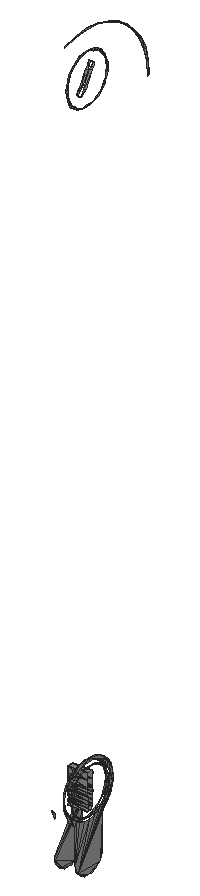
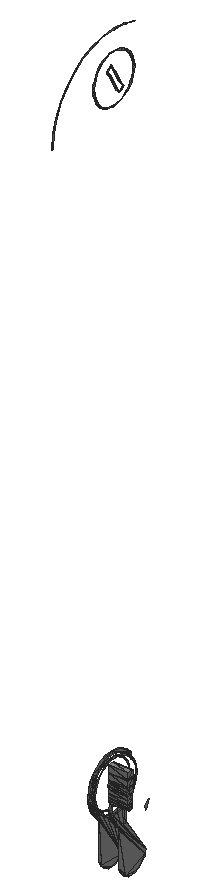
# SketchUp Ruby script. Lengths in inches.
U = 1.inch
M = Sketchup.active_model
def pt(a) = Geom::Point3d.new(a.map { |v| v * U })
def face(e, loops, mat)
  f = e.add_face(loops[0].map { |a| pt(a) })
  loops[1..].each { |l| e.add_face(l.map { |a| pt(a) }).erase! }
  f.material = f.back_material = mat if mat
  f
end
# faces: each face lists its corners as indices into pts; further lists are holes
def faces(e, pts, list, mat = nil) = list.each { |f| face(e, (f[0].is_a?(Array) ? f : [f]).map { |l| l.map { |i| pts[i] } }, mat) }
# xy, xz, yz: faces in a plane at the given z, y or x. An outline is a flat list of corners, or four numbers for a rectangle; further outlines are holes
def ring(l) = l.size == 4 ? [[l[0], l[1]], [l[2], l[1]], [l[2], l[3]], [l[0], l[3]]] : l.each_slice(2).to_a
def flat(e, list, mat, &to3) = list.each { |f| face(e, (f[0].is_a?(Array) ? f : [f]).map { |l| ring(l).map { |u, v| to3.(u, v) } }, mat) }
def xy(e, z, list, mat = nil) = flat(e, list, mat) { |x, y| [x, y, z] }
def xz(e, y, list, mat = nil) = flat(e, list, mat) { |x, z| [x, y, z] }
def yz(e, x, list, mat = nil) = flat(e, list, mat) { |y, z| [x, y, z] }
def lines(e, pts, list) = list.each { |a, b| e.add_line(pt(pts[a]), pt(pts[b])) }
# prism: a flat outline (further loops are holes) pulled along v
def prism(e, loops, v, mat = nil)
  f = face(e, loops, mat); d = Geom::Vector3d.new(v.map { |x| x * U })
  f.pushpull(f.normal.samedirection?(d) ? d.length : -d.length)
end
def box(e, o, s, mat = nil) = prism(e, [[o, [o[0] + s[0], o[1], o[2]], [o[0] + s[0], o[1] + s[1], o[2]], [o[0], o[1] + s[1], o[2]]]], [0, 0, s[2]], mat)
def at(x, y, z, deg = 0) = Geom::Transformation.translation(pt([x, y, z])) * Geom::Transformation.rotation(ORIGIN, Z_AXIS, deg.degrees)
def axes(o, x, y, z) = Geom::Transformation.new([*x, 0, *y, 0, *z, 0, *pt(o).to_a, 1])
def part(name) = M.definitions.add(name)
# library, detail: a bought-in or finely detailed component or shape, given as its bounding box
def library(name, o, s) = part(name).tap { |d| box(d.entities, o, s) }
def detail(e, o, s) = box(e.add_group.entities, o, s)
def put(e, d, t, mat = nil) = e.add_instance(d, t).tap { |i| i.material = mat if mat }
def group(e, t, mat = nil) = e.add_group.tap { |g| g.transformation = t; g.material = mat if mat }.entities
root = M.entities
M.materials.add("Material \#1").color = [140, 140, 140]
xy(root,47.143,[[363.845,397.987,363.845,398.031,364.058,398.031],[363.845,397.987,364.058,398.031,364.058,397.987]],"Material \#1")
xy(root,47.538,[[363.845,397.98,364.058,397.98,363.845,398.053],[364.058,397.98,364.058,398.053,363.845,398.053]],"Material \#1")
xz(root,397.976,[[363.845,47.314,364.058,47.314,363.845,47.342],[364.058,47.314,364.058,47.342,363.845,47.342]],"Material \#1")
xz(root,397.98,[[363.845,47.39,364.058,47.39,363.845,47.454]],"Material \#1")
xz(root,397.987,[[363.845,47.252,364.058,47.252,363.845,47.286],[364.058,47.252,364.058,47.286,363.845,47.286]],"Material \#1")
xz(root,398.046,[[363.845,47.215,363.845,47.252,364.058,47.252]],"Material \#1")
xz(root,398.053,[[363.845,47.473,363.845,47.538,364.058,47.538]],"Material \#1")
yz(root,363.822,[[398.017,46.487,397.932,46.506,397.973,46.492],[398.017,46.487,398.101,46.506,397.932,46.506],[398.017,46.487,398.061,46.492,398.101,46.506],[397.932,46.506,397.829,46.632,397.867,46.557],[397.932,46.506,398.101,46.506,397.829,46.632],
  [398.101,46.506,398.209,47.033,397.829,46.632],[397.932,46.506,397.867,46.557,397.896,46.528],[398.101,46.506,398.137,46.528,398.167,46.557],[398.101,46.506,398.167,46.557,398.204,46.632],[398.101,46.506,398.204,46.632,398.209,47.033],
  [397.867,46.557,397.829,46.632,397.844,46.592],[398.167,46.557,398.19,46.592,398.204,46.632],[397.829,46.632,398.217,47.062,397.824,46.675],[397.829,46.632,398.209,47.033,398.21,47.041],[397.829,46.632,398.21,47.041,398.211,47.048],
  [397.829,46.632,398.211,47.048,398.213,47.055],[397.829,46.632,398.213,47.055,398.217,47.062],[397.824,46.675,398.15,47.075,398.086,47.052],[397.824,46.675,398.207,47.109,398.15,47.075],[397.824,46.675,398.217,47.062,398.254,47.155],
  [397.824,47.033,397.822,47.049,397.824,47.041],[397.822,47.049,397.817,47.062,397.82,47.056],[397.817,47.062,397.827,47.109,397.78,47.155],[398.217,47.062,398.29,47.21,398.254,47.155],[398.217,47.062,398.358,47.296,398.29,47.21],
  [398.226,47.074,398.233,47.08,398.293,47.14],[398.226,47.074,398.293,47.14,398.358,47.296],[398.233,47.08,398.265,47.108,398.293,47.14],[398.293,47.14,398.316,47.175,398.335,47.213],[398.293,47.14,398.335,47.213,398.358,47.296],
  [398.29,47.21,398.358,47.296,398.3125,47.273],[398.3125,47.273,398.358,47.296,398.321,47.34]],"Material \#1")
yz(root,363.845,[[397.987,47.143,398.002,47.173,398.031,47.143],[398.031,47.143,398.002,47.173,398.046,47.173],[398.002,47.173,397.994,47.183,398.046,47.173],[398.046,47.173,397.994,47.183,398.053,47.183],[397.994,47.183,397.994,47.205,398.053,47.183],
  [398.053,47.183,397.994,47.205,398.053,47.205],[397.994,47.205,398.002,47.215,398.053,47.205],[398.053,47.205,398.002,47.215,398.046,47.215],[398.002,47.215,397.987,47.252,398.046,47.215],[398.046,47.215,397.987,47.252,398.046,47.252],
  [397.987,47.252,397.987,47.286,398.046,47.252],[398.046,47.252,397.987,47.286,398.046,47.286],[397.987,47.286,397.976,47.314,398.046,47.286],[398.046,47.286,397.976,47.314,398.057,47.314],[397.976,47.314,397.976,47.342,398.057,47.314],
  [398.057,47.314,397.976,47.342,398.057,47.342],[397.976,47.342,397.987,47.37,398.057,47.342],[398.057,47.342,397.987,47.37,398.046,47.37],[397.987,47.37,397.98,47.39,398.046,47.37],[398.046,47.37,397.98,47.39,398.053,47.39],
  [397.98,47.39,397.98,47.454,398.053,47.39],[398.053,47.39,397.98,47.454,398.053,47.454],[397.98,47.454,397.989,47.459,398.053,47.454],[398.053,47.454,397.989,47.459,398.044,47.459],[397.989,47.459,397.989,47.469,398.044,47.459],
  [398.044,47.459,397.989,47.469,398.044,47.469],[397.989,47.469,397.98,47.473,398.044,47.469],[398.044,47.469,397.98,47.473,398.053,47.473],[397.98,47.473,397.98,47.538,398.053,47.473],[398.053,47.473,397.98,47.538,398.053,47.538]],"Material \#1")
yz(root,364.005,[[398.017,47.044,397.938,47.055,397.941,47.064],[398.017,47.044,397.941,47.064,398.017,47.054],[398.017,47.044,398.017,47.054,398.095,47.055],[398.017,47.054,398.093,47.064,398.095,47.055],[397.938,47.055,397.865,47.084,397.87,47.093],
  [397.938,47.055,397.87,47.093,397.941,47.064],[398.095,47.055,398.093,47.064,398.169,47.084],[398.093,47.064,398.164,47.093,398.169,47.084],[397.865,47.084,397.802,47.131,397.809,47.138],[397.865,47.084,397.809,47.138,397.87,47.093],
  [398.169,47.084,398.164,47.093,398.232,47.131],[398.164,47.093,398.224,47.138,398.232,47.131],[397.802,47.131,397.754,47.192,397.763,47.197],[397.802,47.131,397.763,47.197,397.809,47.138],[398.232,47.131,398.224,47.138,398.28,47.192],
  [398.224,47.138,398.271,47.197,398.28,47.192],[397.754,47.192,397.723,47.264,397.733,47.266],[397.754,47.192,397.733,47.266,397.763,47.197],[398.28,47.192,398.271,47.197,398.31,47.264],[398.271,47.197,398.3,47.266,398.31,47.264],
  [397.723,47.264,397.713,47.34,397.723,47.34],[397.723,47.264,397.723,47.34,397.733,47.266],[398.31,47.264,398.3,47.266,398.321,47.34],[398.3,47.266,398.31,47.34,398.321,47.34],[397.713,47.34,397.723,47.417,397.733,47.414],
  [397.713,47.34,397.733,47.414,397.723,47.34],[398.31,47.34,398.3,47.414,398.31,47.417],[398.31,47.34,398.31,47.417,398.321,47.34],[397.733,47.414,397.723,47.417,397.763,47.483],[398.3,47.414,398.271,47.483,398.28,47.488],
  [398.3,47.414,398.28,47.488,398.31,47.417],[397.723,47.417,397.754,47.488,397.763,47.483],[397.763,47.483,397.754,47.488,397.809,47.542],[398.271,47.483,398.224,47.542,398.232,47.55],[398.271,47.483,398.232,47.55,398.28,47.488],
  [397.754,47.488,397.802,47.55,397.809,47.542],[397.809,47.542,397.802,47.55,397.87,47.588],[398.224,47.542,398.164,47.588,398.169,47.597],[398.224,47.542,398.169,47.597,398.232,47.55],[397.802,47.55,397.865,47.597,397.87,47.588],
  [397.87,47.588,397.865,47.597,397.941,47.617],[398.164,47.588,398.093,47.617,398.095,47.626],[398.164,47.588,398.095,47.626,398.169,47.597],[397.865,47.597,397.938,47.626,397.941,47.617],[397.941,47.617,397.938,47.626,398.017,47.626],
  [398.093,47.617,398.017,47.626,398.017,47.636],[398.093,47.617,398.017,47.636,398.095,47.626],[397.938,47.626,398.017,47.636,398.017,47.626]],"Material \#1")
yz(root,364.028,[[398.888,54.238,398.873,54.397,398.888,54.399],[398.888,54.238,398.888,54.399,398.903,54.239],[398.017,54.303,397.964,54.307,397.967,54.322],[398.017,54.303,397.967,54.322,398.017,54.318],[398.017,54.303,398.017,54.318,398.069,54.307],
  [397.964,54.307,397.914,54.321,397.92,54.335],[397.964,54.307,397.92,54.335,397.967,54.322],[398.069,54.307,398.017,54.318,398.067,54.322],[398.069,54.307,398.067,54.322,398.119,54.321],[397.914,54.321,397.868,54.342,397.876,54.355],
  [397.914,54.321,397.876,54.355,397.92,54.335],[398.119,54.321,398.067,54.322,398.114,54.335],[398.119,54.321,398.114,54.335,398.165,54.342],[398.114,54.335,398.158,54.355,398.165,54.342],[397.868,54.342,397.827,54.37,397.837,54.382],
  [397.868,54.342,397.837,54.382,397.876,54.355],[398.165,54.342,398.158,54.355,398.206,54.37],[398.158,54.355,398.197,54.382,398.206,54.37],[397.827,54.37,397.792,54.405,397.803,54.414],[397.827,54.37,397.803,54.414,397.837,54.382],
  [398.206,54.37,398.197,54.382,398.242,54.405],[398.197,54.382,398.23,54.414,398.242,54.405],[398.873,54.397,398.833,54.54,398.847,54.545],[398.873,54.397,398.847,54.545,398.888,54.399],[397.792,54.405,397.763,54.445,397.776,54.452],
  [397.792,54.405,397.776,54.452,397.803,54.414],[398.242,54.405,398.23,54.414,398.271,54.445],[398.23,54.414,398.258,54.452,398.271,54.445],[397.763,54.445,397.741,54.489,397.755,54.495],[397.763,54.445,397.755,54.495,397.776,54.452],
  [398.271,54.445,398.258,54.452,398.293,54.489],[398.258,54.452,398.278,54.495,398.293,54.489],[397.741,54.489,397.727,54.538,397.742,54.541],[397.741,54.489,397.742,54.541,397.755,54.495],[398.293,54.489,398.278,54.495,398.306,54.538],
  [398.278,54.495,398.291,54.541,398.306,54.538],[397.727,54.538,397.723,54.589,397.738,54.589],[397.727,54.538,397.738,54.589,397.742,54.541],[398.306,54.538,398.291,54.541,398.311,54.603],[398.833,54.54,398.768,54.672,398.781,54.679],
  [398.833,54.54,398.781,54.679,398.847,54.545],[398.291,54.541,398.296,54.602,398.311,54.603],[397.723,54.589,397.727,54.641,397.742,54.638],[397.723,54.589,397.742,54.638,397.738,54.589],[398.296,54.602,398.291,54.638,398.306,54.641],
  [398.296,54.602,398.306,54.641,398.311,54.603],[397.742,54.638,397.727,54.641,397.755,54.684],[398.291,54.638,398.278,54.684,398.293,54.689],[398.291,54.638,398.293,54.689,398.306,54.641],[397.727,54.641,397.741,54.689,397.755,54.684],
  [398.768,54.672,398.679,54.794,398.69,54.804],[398.768,54.672,398.69,54.804,398.781,54.679],[397.755,54.684,397.741,54.689,397.776,54.726],[398.278,54.684,398.258,54.726,398.271,54.734],[398.278,54.684,398.271,54.734,398.293,54.689],
  [397.741,54.689,397.763,54.734,397.776,54.726],[397.776,54.726,397.763,54.734,397.803,54.764],[398.258,54.726,398.23,54.764,398.242,54.774],[398.258,54.726,398.242,54.774,398.271,54.734],[397.763,54.734,397.792,54.774,397.803,54.764],
  [397.803,54.764,397.792,54.774,397.837,54.797],[398.23,54.764,398.197,54.797,398.206,54.808],[398.23,54.764,398.206,54.808,398.242,54.774],[397.792,54.774,397.827,54.808,397.837,54.797],[398.679,54.794,398.577,54.892,398.587,54.904],
  [398.679,54.794,398.587,54.904,398.69,54.804],[397.837,54.797,397.827,54.808,397.876,54.824],[398.197,54.797,398.158,54.824,398.165,54.837],[398.197,54.797,398.165,54.837,398.206,54.808],[397.827,54.808,397.868,54.837,397.876,54.824],
  [397.876,54.824,397.868,54.837,397.92,54.844],[398.158,54.824,398.114,54.844,398.119,54.858],[398.158,54.824,398.119,54.858,398.165,54.837],[397.868,54.837,397.914,54.858,397.92,54.844],[397.92,54.844,397.914,54.858,397.967,54.857],
  [398.114,54.844,398.067,54.857,398.069,54.871],[398.114,54.844,398.069,54.871,398.119,54.858],[397.967,54.857,397.914,54.858,397.964,54.871],[397.967,54.857,397.964,54.871,398.017,54.861],[398.067,54.857,398.017,54.861,398.017,54.876],
  [398.067,54.857,398.017,54.876,398.069,54.871],[398.017,54.861,397.964,54.871,398.017,54.876],[398.577,54.892,398.456,54.976,398.464,54.989],[398.577,54.892,398.464,54.989,398.587,54.904],[398.456,54.976,398.32,55.039,398.326,55.053],
  [398.456,54.976,398.326,55.053,398.464,54.989],[397.713,55.039,397.708,55.053,397.86,55.078],[398.32,55.039,398.173,55.078,398.176,55.093],[398.32,55.039,398.176,55.093,398.326,55.053],[397.708,55.053,397.858,55.093,397.86,55.078],
  [397.86,55.078,397.858,55.093,398.017,55.092],[398.173,55.078,398.017,55.092,398.017,55.107],[398.173,55.078,398.017,55.107,398.176,55.093],[398.017,55.092,397.858,55.093,398.017,55.107]],"Material \#1")
yz(root,364.051,[[398.017,46.487,397.867,46.557,398.167,46.557],[398.017,46.487,397.932,46.506,397.867,46.557],[398.017,46.487,397.973,46.492,397.932,46.506],[398.017,46.487,398.101,46.506,398.061,46.492],[398.017,46.487,398.167,46.557,398.101,46.506],
  [397.932,46.506,397.896,46.528,397.867,46.557],[398.101,46.506,398.167,46.557,398.137,46.528],[397.867,46.557,397.824,46.675,398.017,47.044],[397.867,46.557,397.829,46.632,397.824,46.675],[397.867,46.557,397.844,46.592,397.829,46.632],
  [397.867,46.557,398.017,47.044,398.086,47.052],[397.867,46.557,398.086,47.052,398.15,47.075],[397.867,46.557,398.15,47.075,398.207,47.109],[397.867,46.557,398.207,47.109,398.254,47.155],[397.867,46.557,398.21,47.041,398.167,46.557],
  [397.867,46.557,398.211,47.048,398.21,47.041],[397.867,46.557,398.213,47.055,398.211,47.048],[397.867,46.557,398.217,47.062,398.213,47.055],[397.867,46.557,398.254,47.155,398.358,47.296],[397.867,46.557,398.358,47.296,398.217,47.062],
  [398.167,46.557,398.204,46.632,398.19,46.592],[398.167,46.557,398.209,47.033,398.204,46.632],[398.167,46.557,398.21,47.041,398.209,47.033],[398.204,46.632,398.209,47.033,398.209,46.675],[397.824,46.675,397.824,47.033,397.827,47.109],
  [397.824,46.675,397.827,47.109,397.883,47.075],[397.824,46.675,397.883,47.075,397.947,47.052],[397.824,46.675,397.947,47.052,398.017,47.044],[397.824,47.033,397.822,47.049,397.827,47.109],[397.824,47.033,397.824,47.041,397.822,47.049],
  [397.822,47.049,397.78,47.155,397.827,47.109],[397.822,47.049,397.817,47.062,397.78,47.155],[397.822,47.049,397.82,47.056,397.817,47.062],[397.817,47.062,397.676,47.296,397.744,47.21],[397.817,47.062,397.812,47.068,397.676,47.296],
  [397.817,47.062,397.744,47.21,397.78,47.155],[398.217,47.062,398.358,47.296,398.221,47.068],[397.812,47.068,397.807,47.074,397.676,47.296],[398.221,47.068,398.358,47.296,398.226,47.074],[397.807,47.074,397.742,47.141,397.676,47.296],
  [397.807,47.074,397.801,47.08,397.742,47.141],[398.226,47.074,398.293,47.14,398.233,47.08],[398.226,47.074,398.358,47.296,398.293,47.14],[397.801,47.08,397.77,47.109,397.742,47.141],[398.233,47.08,398.293,47.14,398.265,47.108],
  [398.293,47.14,398.335,47.213,398.316,47.175],[398.293,47.14,398.358,47.296,398.335,47.213],[398.254,47.155,398.29,47.21,398.358,47.296],[398.29,47.21,398.3125,47.273,398.358,47.296],[398.335,47.213,398.358,47.296,398.349,47.253],
  [398.3125,47.273,398.321,47.34,398.358,47.296],[398.358,47.296,398.285,47.55,398.352,47.417],[398.358,47.296,398.3125,47.408,398.285,47.55],[398.358,47.296,398.321,47.34,398.3125,47.408],[398.358,47.296,398.352,47.417,398.361,47.34],
  [398.3125,47.408,398.29,47.47,398.285,47.55],[398.352,47.417,398.285,47.55,398.326,47.488],[397.744,47.47,397.748,47.55,397.78,47.525],[398.29,47.47,398.254,47.525,398.285,47.55],[397.78,47.525,397.748,47.55,397.827,47.571],
  [398.254,47.525,398.207,47.571,398.285,47.55],[397.748,47.55,397.801,47.602,397.865,47.642],[397.748,47.55,397.865,47.642,398.017,47.676],[397.748,47.55,397.883,47.606,397.827,47.571],[397.748,47.55,398.017,47.676,397.883,47.606],
  [398.285,47.55,398.017,47.676,398.168,47.642],[398.285,47.55,398.15,47.606,398.017,47.676],[398.285,47.55,398.207,47.571,398.15,47.606],[398.285,47.55,398.168,47.642,398.232,47.602],[397.883,47.606,398.017,47.676,397.947,47.628],
  [398.15,47.606,398.086,47.628,398.017,47.676],[397.947,47.628,398.017,47.676,398.017,47.636],[398.086,47.628,398.017,47.636,398.017,47.676],[397.865,47.642,397.938,47.667,398.017,47.676],[398.168,47.642,398.017,47.676,398.096,47.667]],"Material \#1")
yz(root,364.058,[[398.017,47.077,397.947,47.086,397.949,47.095],[398.017,47.077,397.949,47.095,398.017,47.087],[398.017,47.077,398.017,47.087,398.087,47.086],[397.947,47.086,397.881,47.112,397.887,47.121],[397.947,47.086,397.887,47.121,397.949,47.095],
  [398.087,47.086,398.017,47.087,398.084,47.095],[398.087,47.086,398.084,47.095,398.152,47.112],[398.084,47.095,398.147,47.121,398.152,47.112],[397.881,47.112,397.825,47.154,397.833,47.161],[397.881,47.112,397.833,47.161,397.887,47.121],
  [398.152,47.112,398.147,47.121,398.208,47.154],[398.147,47.121,398.201,47.161,398.208,47.154],[397.825,47.154,397.782,47.208,397.791,47.213],[397.825,47.154,397.791,47.213,397.833,47.161],[398.208,47.154,398.201,47.161,398.251,47.208],
  [398.201,47.161,398.242,47.213,398.251,47.208],[397.782,47.208,397.755,47.272,397.765,47.275],[397.782,47.208,397.765,47.275,397.791,47.213],[398.251,47.208,398.242,47.213,398.278,47.272],[398.242,47.213,398.268,47.275,398.278,47.272],
  [397.755,47.272,397.746,47.34,397.756,47.34],[397.755,47.272,397.756,47.34,397.765,47.275],[398.278,47.272,398.268,47.275,398.288,47.34],[398.268,47.275,398.277,47.34,398.288,47.34],[397.746,47.34,397.755,47.409,397.765,47.406],
  [397.746,47.34,397.765,47.406,397.756,47.34],[398.277,47.34,398.268,47.406,398.278,47.409],[398.277,47.34,398.278,47.409,398.288,47.34],[397.765,47.406,397.755,47.409,397.791,47.467],[398.268,47.406,398.242,47.467,398.251,47.472],
  [398.268,47.406,398.251,47.472,398.278,47.409],[397.755,47.409,397.782,47.472,397.791,47.467],[397.791,47.467,397.782,47.472,397.833,47.52],[398.242,47.467,398.201,47.52,398.208,47.527],[398.242,47.467,398.208,47.527,398.251,47.472],
  [397.782,47.472,397.825,47.527,397.833,47.52],[397.833,47.52,397.825,47.527,397.887,47.56],[398.201,47.52,398.147,47.56,398.152,47.569],[398.201,47.52,398.152,47.569,398.208,47.527],[397.825,47.527,397.881,47.569,397.887,47.56],
  [397.887,47.56,397.881,47.569,397.949,47.585],[398.147,47.56,398.084,47.585,398.087,47.595],[398.147,47.56,398.087,47.595,398.152,47.569],[397.881,47.569,397.947,47.595,397.949,47.585],[397.949,47.585,397.947,47.595,398.017,47.594],
  [398.084,47.585,398.017,47.594,398.017,47.604],[398.084,47.585,398.017,47.604,398.087,47.595],[398.017,47.594,397.947,47.595,398.017,47.604]],"Material \#1")
p = [[364.058,398.05,47.178],[364.058,398.031,47.143],[363.845,398.031,47.143],[363.845,398.046,47.173],[364.058,398.05,47.178],[363.845,398.002,47.173],
  [363.845,397.987,47.143],[364.058,397.987,47.143],[364.058,397.987,47.143],[364.058,397.998,47.178],[363.845,398.002,47.173],[363.845,397.987,47.252],
  [363.845,398.002,47.215],[364.058,397.998,47.21],[364.058,397.998,47.21],[363.845,398.002,47.215],[363.845,397.994,47.205],[364.058,397.998,47.178],
  [363.845,397.994,47.183],[363.845,398.002,47.173],[364.058,398.05,47.21],[363.845,398.053,47.205],[363.845,398.046,47.215],[364.058,398.05,47.178],
  [363.845,398.046,47.173],[363.845,398.053,47.183],[364.058,397.998,47.178],[364.058,397.998,47.21],[363.845,397.994,47.205],[363.845,397.994,47.183],
  [364.058,398.05,47.21],[364.058,398.05,47.178],[363.845,398.053,47.183],[363.845,398.053,47.205],[364.058,397.998,47.21],[364.058,397.987,47.252],
  [363.845,397.987,47.252],[364.058,398.046,47.252],[364.058,398.05,47.21],[363.845,398.046,47.215],[363.845,397.987,47.37],[363.845,397.976,47.342],
  [364.058,397.976,47.342],[363.845,398.057,47.342],[363.845,398.046,47.37],[364.058,398.049,47.38],[363.845,398.046,47.286],[363.845,398.057,47.314],
  [364.058,398.057,47.328],[363.845,398.046,47.252],[363.845,398.046,47.286],[364.058,398.051,47.3],[364.058,397.987,47.286],[364.058,397.976,47.314],
  [363.845,397.976,47.314],[363.845,397.987,47.286],[364.058,397.976,47.342],[364.058,397.987,47.37],[363.845,397.987,47.37],[364.058,398.049,47.38],
  [364.058,398.051,47.356],[363.845,398.057,47.342],[364.058,398.057,47.328],[364.058,398.051,47.3],[363.845,398.046,47.286],[364.058,398.051,47.3],
  [364.058,398.046,47.252],[363.845,398.046,47.252],[363.845,398.057,47.314],[363.845,398.057,47.342],[364.058,398.051,47.356],[364.058,398.051,47.356],
  [364.058,398.057,47.328],[363.845,398.057,47.314],[363.845,397.98,47.39],[363.845,397.987,47.37],[364.058,397.987,47.37],[363.845,398.053,47.39],
  [363.845,398.053,47.454],[364.058,398.05,47.459],[363.845,398.046,47.37],[363.845,398.053,47.39],[364.058,398.053,47.394],[364.058,397.987,47.37],
  [364.058,397.98,47.39],[363.845,397.98,47.39],[364.058,397.98,47.39],[364.058,397.984,47.466],[363.845,397.98,47.454],[364.058,398.05,47.459],
  [364.058,398.053,47.394],[363.845,398.053,47.39],[364.058,398.053,47.394],[364.058,398.049,47.38],[363.845,398.046,47.37],[364.058,397.984,47.466],
  [363.845,397.989,47.459],[363.845,397.98,47.454],[364.058,398.05,47.459],[363.845,398.044,47.459],[363.845,398.044,47.469],[364.058,398.05,47.459],
  [363.845,398.053,47.473],[364.058,398.05,47.459],[363.845,398.053,47.454],[364.058,397.984,47.466],[363.845,397.98,47.473],[363.845,397.989,47.469],
  [364.058,397.984,47.466],[363.845,397.98,47.538],[363.845,397.98,47.473],[364.058,397.984,47.466],[364.058,397.984,47.466],[364.058,397.98,47.538],
  [363.845,397.98,47.538],[364.058,398.053,47.538],[364.058,398.05,47.459],[363.845,398.053,47.473],[364.024,397.963,54.432],[364.024,397.931,54.445],
  [364.005,397.931,54.445],[364.005,397.963,54.432],[364.024,397.903,54.466],[364.005,397.903,54.466],[364.029,397.982,54.465],[364.01,397.982,54.465],
  [364.029,397.923,54.498],[364.01,397.923,54.498],[364.031,397.94,54.527],[364.012,397.94,54.527],[364.031,398.034,54.685],[364.012,398.034,54.685],
  [364.031,398.093,54.652],[364.031,398,54.494],[364.012,398,54.494],[364.012,398.093,54.652],[364.029,398.051,54.714],[364.01,398.051,54.714],
  [364.024,398.07,54.747],[364.005,398.07,54.747],[364.024,398.102,54.734],[364.005,398.102,54.734],[364.024,398.13,54.713],[364.005,398.13,54.713],
  [364.029,398.111,54.681],[364.01,398.111,54.681],[546.148,444.956,116.713],[546.148,445.552,115.686]]
faces(root,p,[[0,1,2],[2,3,4],[5,6,7],[8,9,10],[11,12,13],[14,15,16],[17,18,19],[20,21,22],
  [23,24,25],[26,27,28],[28,29,26],[30,31,32],[32,33,30],[34,35,36],[37,38,39],[40,41,42],
  [43,44,45],[46,47,48],[49,50,51],[52,53,54],[54,55,52],[56,57,58],[59,60,61],[62,63,64],
  [65,66,67],[68,69,70],[71,72,73],[74,75,76],[77,78,79],[80,81,82],[83,84,85],[86,87,88],
  [89,90,91],[92,93,94],[95,96,97],[98,99,100],[101,100,102],[103,104,99],[105,106,107],[108,107,96],
  [109,110,111],[112,113,114],[115,116,117],[118,119,120],[120,121,118],[119,122,123],[123,120,119],[124,118,121],
  [121,125,124],[122,126,127],[127,123,122],[126,128,129],[129,127,126],[128,130,131],[131,129,128],[132,133,134],
  [134,135,132],[133,124,125],[125,134,133],[130,136,137],[137,131,130],[136,138,139],[139,137,136],[138,140,141],
  [141,139,138],[140,142,143],[143,141,140],[142,144,145],[145,143,142],[144,132,135],[135,145,144]],"Material \#1")
lines(root,p,[[146,147]])
